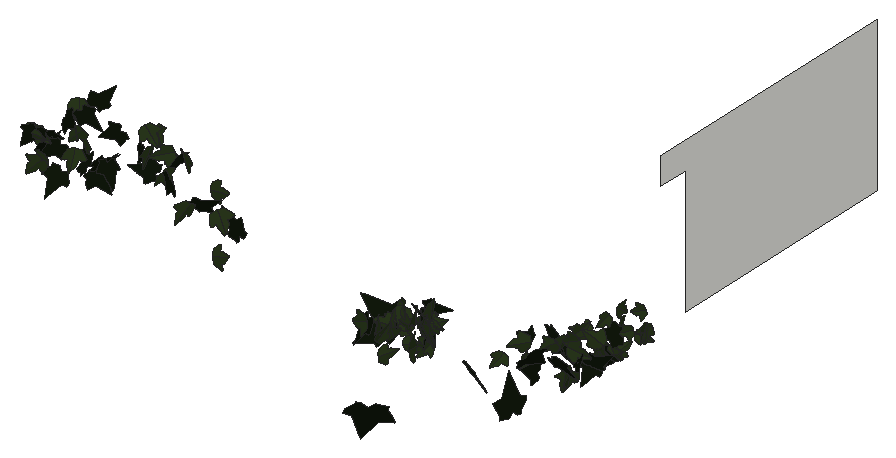
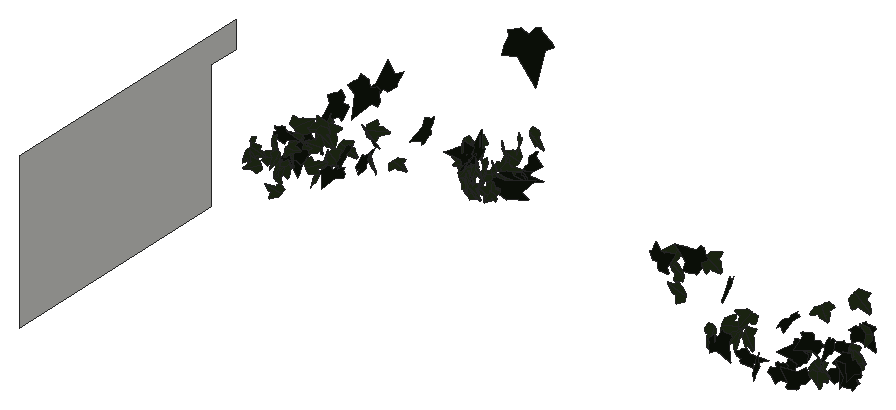
# SketchUp Ruby script. Lengths in inches.
U = 1.inch
M = Sketchup.active_model
def pt(a) = Geom::Point3d.new(a.map { |v| v * U })
def face(e, loops, mat)
  f = e.add_face(loops[0].map { |a| pt(a) })
  loops[1..].each { |l| e.add_face(l.map { |a| pt(a) }).erase! }
  f.material = f.back_material = mat if mat
  f
end
# faces: each face lists its corners as indices into pts; further lists are holes
def faces(e, pts, list, mat = nil) = list.each { |f| face(e, (f[0].is_a?(Array) ? f : [f]).map { |l| l.map { |i| pts[i] } }, mat) }
# xy, xz, yz: faces in a plane at the given z, y or x. An outline is a flat list of corners, or four numbers for a rectangle; further outlines are holes
def ring(l) = l.size == 4 ? [[l[0], l[1]], [l[2], l[1]], [l[2], l[3]], [l[0], l[3]]] : l.each_slice(2).to_a
def flat(e, list, mat, &to3) = list.each { |f| face(e, (f[0].is_a?(Array) ? f : [f]).map { |l| ring(l).map { |u, v| to3.(u, v) } }, mat) }
def xy(e, z, list, mat = nil) = flat(e, list, mat) { |x, y| [x, y, z] }
def xz(e, y, list, mat = nil) = flat(e, list, mat) { |x, z| [x, y, z] }
def yz(e, x, list, mat = nil) = flat(e, list, mat) { |y, z| [x, y, z] }
def lines(e, pts, list) = list.each { |a, b| e.add_line(pt(pts[a]), pt(pts[b])) }
# prism: a flat outline (further loops are holes) pulled along v
def prism(e, loops, v, mat = nil)
  f = face(e, loops, mat); d = Geom::Vector3d.new(v.map { |x| x * U })
  f.pushpull(f.normal.samedirection?(d) ? d.length : -d.length)
end
def box(e, o, s, mat = nil) = prism(e, [[o, [o[0] + s[0], o[1], o[2]], [o[0] + s[0], o[1] + s[1], o[2]], [o[0], o[1] + s[1], o[2]]]], [0, 0, s[2]], mat)
def at(x, y, z, deg = 0) = Geom::Transformation.translation(pt([x, y, z])) * Geom::Transformation.rotation(ORIGIN, Z_AXIS, deg.degrees)
def axes(o, x, y, z) = Geom::Transformation.new([*x, 0, *y, 0, *z, 0, *pt(o).to_a, 1])
def part(name) = M.definitions.add(name)
# library, detail: a bought-in or finely detailed component or shape, given as its bounding box
def library(name, o, s) = part(name).tap { |d| box(d.entities, o, s) }
def detail(e, o, s) = box(e.add_group.entities, o, s)
def put(e, d, t, mat = nil) = e.add_instance(d, t).tap { |i| i.material = mat if mat }
def group(e, t, mat = nil) = e.add_group.tap { |g| g.transformation = t; g.material = mat if mat }.entities
root = M.entities
M.materials.add("efeu1").color = [18, 25, 13]
M.materials.add("efeu2").color = [43, 57, 29]
c1 = part("ivyleaf_10")
p = [[0,0.5,-0.03],[-0.0625,2.02,-0.43],[-0.19,2.01,-0.46],[-0.54,1.05,-0.29],[-0.52,0.625,-0.18],[-0.83,0.76,-0.28],
  [-1.16,0.64,-0.33],[-1.15,0.33,-0.24],[-0.77,-0.39,0.02],[-0.3,-0.51,0.16],[0.04,-0.48,0.23],[-0.02,2.01,-0.4375],
  [-0.06,2.01,-0.43],[0.04,-0.49,0.23],[0.67,-0.49,0.14],[1.38,0.36,-0.2],[1.375,0.51,-0.24],[0.81,0.65,-0.19],
  [0.62,0.59,-0.15],[0.6,1.09,-0.28],[0.5,1.23,-0.31]]
faces(c1.entities,p,[[0,1,2,3,4,5,6,7,8,9,10],[11,12,0,13,14,15,16,17,18,19,20]],"efeu2")
c2 = part("ivyleaf_9")
p = [[1.54,2.16,1.25],[1.36,2.04,1.19],[-0.21,0.99,0.68],[-0.71,1.11,0.82],[-0.85,0.86,0.67],[-0.8,0.17,0.21],
  [-0.9,-0.01,0.1],[-0.67,-0.16,-0.02],[-0.08,-0.08,-0.05],[-0.03,-0.6,-0.4],[0.65,-0.88,-0.66],[0.83,-0.6,-0.49],
  [1.29,-0.42,-0.43],[1.8125,-0.07,-0.26],[1.21,0.44,0.15]]
faces(c2.entities,p,[[0,1,2,3,4,5,6,7,8,9,10,11,12,13,14]],"efeu1")
p = [[600,172.6875,154.12],[600,172.6875,171.1],[600.49,142.28,171.1],[600.49,142.28,168.16],[600.44,145.72,168.16],[600.44,145.72,154.12]]
faces(root,p,[[0,1,2,3,4,5]])
put(root,c1,axes([538.16,133.79,155.21],[0.18163,0.01122,0.75224],[0.73526,0.16121,-0.17993],[-0.1593,0.75687,0.02717]))
put(root,c2,axes([538.4,134.09,153.71],[0.30381,0.77459,-0.0565],[-0.01137,0.06509,0.83133],[0.77656,-0.30209,0.03427]))
put(root,c1,axes([538.64,138.9,156.16],[0.7212,0.27698,0.03221],[0.02999,0.01177,-0.77256],[-0.27723,0.72182,0.00023]))
put(root,c2,axes([538.86,134.06,155.24],[0.69763,0.51598,-0.17397],[-0.14038,-0.10277,-0.86772],[-0.52612,0.71162,0.00083]))
put(root,c2,axes([539.65,131.65,157.125],[0.19614,0.36038,-0.73019],[-0.34317,-0.64453,-0.41029],[-0.73844,0.39526,-0.00328]))
put(root,c2,axes([539.93,134.62,154.3],[0.02323,0.06156,-0.80436],[-0.30244,-0.74534,-0.06577],[-0.74788,0.30332,0.00162]))
put(root,c1,axes([539.03,131.61,156.8],[-0.18917,0.06706,-0.77238],[0.75356,-0.17103,-0.1994],[-0.18229,-0.7766,-0.02279]))
put(root,c2,axes([539.55,140.36,155.67],[-0.19047,-0.10209,0.79318],[0.77188,0.18982,0.20979],[-0.2092,0.79334,0.05188]))
put(root,c1,axes([540.03,136.89,154.5],[-0.51647,0.40191,0.41635],[0.33105,-0.25253,0.65441],[0.47464,0.61345,-0.00339]))
put(root,c1,axes([540.78,131.4,154.4375],[0.30694,-0.14086,-0.77767],[-0.71473,0.30658,-0.33763],[0.33731,0.77781,-0.00775]))
put(root,c2,axes([540.38,135.1,157],[0.17453,-0.20926,-0.75548],[-0.52984,0.53894,-0.27169],[0.57776,0.55746,-0.02094]))
put(root,c1,axes([540.8125,136.42,155.11],[-0.53976,-0.24221,0.56706],[-0.51907,-0.22834,-0.59161],[0.33286,-0.74884,-0.00302]))
put(root,c2,axes([541.37,136.16,157.42],[-0.0648,-0.13453,-0.80919],[0.55258,0.59275,-0.1428],[0.60625,-0.55465,0.04366]))
put(root,c2,axes([543.28,138.8,155.03],[-0.03916,0.10134,-0.79983],[-0.5954,-0.54355,-0.03972],[-0.54359,0.58805,0.10112]))
put(root,c2,axes([542.9,131,154.14],[-0.68653,-0.5213,-0.0395],[0.03659,0.01712,-0.86198],[0.52152,-0.68746,0.00848]))
put(root,c1,axes([543.51,127.41,157.07],[-0.55173,-0.34553,0.61966],[-0.503,-0.3631,-0.65033],[0.50036,-0.74602,0.02952]))
put(root,c1,axes([543.25,134.12,155.76],[-0.53137,0.47422,-0.42591],[0.30278,-0.30016,-0.71195],[-0.5609,-0.61128,0.01917]))
put(root,c2,axes([544.21,133.08,154.47],[-0.63931,0.2044,-0.45949],[-0.43596,0.14522,0.67118],[0.2507,0.7738,-0.00459]))
put(root,c2,axes([544.41,136.02,153.72],[-0.33925,0.575,-0.45103],[0.20796,-0.40075,-0.66731],[-0.70058,-0.3974,0.02033]))
put(root,c2,axes([544.52,133.79,154.14],[0.05579,0.62679,-0.58324],[-0.04631,0.58583,0.62515],[0.85492,-0.00917,0.07192]))
put(root,c1,axes([544.81,130.57,156.96],[0.56058,0.63253,-0.23032],[-0.15906,-0.16677,-0.84515],[-0.65409,0.58265,0.00813]))
put(root,c2,axes([545.01,133.38,153.82],[0.03779,-0.50189,-0.72315],[-0.05962,0.72069,-0.5033],[0.87823,0.07052,-0.00306]))
put(root,c2,axes([545.875,138.52,154.37],[-0.02382,0.00622,-0.82368],[0.71569,-0.40778,-0.02378],[-0.40777,-0.71606,0.00638]))
put(root,c2,axes([547.1,132.48,155.89],[0.04586,-0.77951,-0.22466],[-0.01365,0.22425,-0.78086],[0.81112,0.04784,-0.00044]))
put(root,c1,axes([547.72,138.49,156.72],[-0.15617,0.81876,0.06978],[-0.01288,0.06859,-0.83352],[-0.82162,-0.1567,-0.0002]))
put(root,c2,axes([548.48,137,153.48],[-0.38187,0.07115,0.73811],[-0.72908,0.11553,-0.38833],[-0.13536,-0.82298,0.0093]))
put(root,c1,axes([548.23,136.72,155.76],[0.12811,-0.82101,0.27076],[0.07379,-0.26233,-0.83037],[0.86135,0.14458,0.03086]))
put(root,c1,axes([548.08,136.63,157.75],[0.59729,0.41037,0.48709],[0.37733,0.30997,-0.72385],[-0.51311,0.70564,0.03469]))
put(root,c1,axes([550.34,136.91,156.13],[0.16305,0.08602,-0.82421],[-0.70824,-0.42167,-0.18411],[-0.43025,0.72671,-0.00927]))
put(root,c2,axes([550.38,138,155.27],[-0.07722,0.63035,-0.56912],[0.09084,-0.56206,-0.63485],[-0.84438,-0.11811,-0.01626]))
put(root,c1,axes([550.95,135.43,154.9],[-0.31424,-0.69836,-0.44569],[0.19447,0.40118,-0.76573],[0.80532,-0.36938,0.01099]))
put(root,c1,axes([551.18,137.97,155.75],[-0.7459,0.42304,-0.01831],[0.01592,-0.00904,-0.85751],[-0.42314,-0.74607,0.00001]))
put(root,c2,axes([553.61,132.75,156.47],[0.4271,-0.24571,-0.70668],[0.60894,-0.35862,0.49272],[-0.4347,-0.74378,-0.00412]))
put(root,c1,axes([557.17,134.7,155.82],[0.12973,-0.0419,-0.87246],[0.81019,-0.32381,0.13602],[-0.32638,-0.82046,-0.00913]))
put(root,c1,axes([558.06,129.68,156.66],[-0.22354,-0.67295,0.54403],[-0.10724,-0.53601,-0.70709],[0.85867,-0.24213,0.05332]))
put(root,c2,axes([558.53,130.5,156.67],[0.64407,0.48312,-0.40607],[0.32501,0.24344,0.80513],[0.54099,-0.72143,-0.00025]))
put(root,c1,axes([561.23,130.13,156.78],[0.52281,0.70498,0.2678],[0.16092,0.21407,-0.87768],[-0.73676,0.54701,-0.00166]))
put(root,c2,axes([562.92,130.68,155.23],[0.0634,-0.10933,0.99298],[-0.68294,0.72142,0.12303],[-0.72908,-0.68527,-0.0289]))
put(root,c1,axes([562.01,128.83,153.5],[0.28453,-0.18791,-0.84865],[0.74938,-0.39941,0.33969],[-0.4404,-0.80103,0.02971]))
put(root,c2,axes([582.43,127.95,154.38],[-1.0884,-0.64831,-0.54177],[-0.43949,-0.32015,1.26602],[-0.72158,1.17288,0.0461]))
put(root,c2,axes([581.74,125.07,155.83],[-0.02417,-0.01205,-0.91198],[0.56003,-0.72025,-0.00532],[-0.71987,-0.55993,0.02647]))
put(root,c2,axes([582.35,125.81,154.49],[-0.59916,-0.32383,0.4931],[-0.42255,-0.25486,-0.68081],[0.41165,-0.73293,0.01887]))
put(root,c2,axes([583.1,126.6,154.76],[-0.5473,0.0676,0.53336],[-0.53523,0.0033,-0.54963],[-0.05073,-0.7642,0.04481]))
put(root,c1,axes([582.99,126.52,155.14],[0.14239,0.17184,0.74485],[-0.56321,-0.4887,0.22041],[0.51685,-0.57987,0.03498]))
put(root,c1,axes([583.14,122.71,157.2],[0.32433,-0.22794,-0.81599],[-0.67575,0.45743,-0.39637],[0.51104,0.74952,-0.00626]))
put(root,c1,axes([582.91,128.51,155.63],[0.61668,0.31527,-0.16842],[-0.15247,-0.07174,-0.69258],[-0.32328,0.63523,0.00537]))
put(root,c1,axes([582.67,128.54,156.21],[0.39763,-0.1483,0.61159],[0.57181,-0.21699,-0.42437],[0.26281,0.69646,-0.00199]))
put(root,c1,axes([583.14,128.62,154.11],[0.63031,0.27778,0.07534],[-0.07011,-0.02772,0.6888],[0.27915,-0.63419,0.00289]))
put(root,c1,axes([584,127.84,154.95],[-0.07099,-0.01051,0.63782],[-0.63754,0.02298,-0.07058],[-0.02168,-0.64134,-0.01299]))
put(root,c1,axes([583.2,128.58,153.99],[0.54948,0.03532,0.39755],[0.39654,0.02841,-0.55061],[-0.04527,0.67762,0.00236]))
put(root,c1,axes([583.68,124.12,156.7],[-0.04347,0.20265,-0.74578],[0.20959,-0.71587,-0.20674],[-0.74386,-0.21355,-0.01467]))
put(root,c1,axes([583.86,124.21,155.14],[0.01918,-0.59675,0.48372],[-0.02502,0.48313,0.59701],[-0.76777,-0.03065,-0.00737]))
put(root,c1,axes([584.06,125.75,154.84],[-0.24294,-0.54044,-0.26284],[-0.10862,-0.23935,0.59253],[-0.59107,0.26611,-0.00086]))
put(root,c1,axes([583.93,125.62,156.16],[0.46115,-0.45321,-0.14519],[0.10334,-0.10198,0.64657],[-0.46454,-0.47258,-0.00029]))
put(root,c1,axes([584.01,124.29,153.46],[0.04693,0.03629,-0.77118],[0.48642,0.59857,0.05777],[0.59952,-0.4885,0.01349]))
put(root,c1,axes([583.98,127.6875,153.0625],[0.18511,-0.01668,-0.62513],[0.62378,-0.04121,0.18581],[-0.04425,-0.65065,0.00425]))
put(root,c1,axes([585.65,128.02,155.49],[-0.15905,0.07464,0.7275],[-0.72612,0.07245,-0.16619],[-0.087,-0.74115,0.05702]))
put(root,c1,axes([585.32,128.61,155.57],[0.08297,0.81543,0.03993],[0.00051,0.04008,-0.81964],[-0.81641,0.08289,0.00354]))
put(root,c1,axes([585.74,128.16,152.92],[-0.2941,-0.21841,-0.59072],[-0.43307,-0.40324,0.3647],[-0.45728,0.52235,0.03453]))
put(root,c1,axes([585.67,128.5,155.34],[-0.13623,-0.6718,0.17915],[-0.03624,-0.17545,-0.68547],[0.69433,-0.14096,-0.00063]))
put(root,c1,axes([585.78,128.86,154.98],[0.32065,-0.5272,-0.54501],[-0.24253,0.48934,-0.61604],[0.71844,0.40049,0.03529]))
put(root,c1,axes([586,128.2,153.57],[0.57919,-0.07349,-0.5641],[-0.56073,0.06187,-0.58379],[0.09584,0.80612,-0.00662]))
put(root,c2,axes([585.51,127.77,156.46],[0.68865,-0.41895,0.0137],[-0.00933,0.01102,0.80606],[-0.41907,-0.68869,0.00457]))
put(root,c1,axes([585.79,128.8,154.26],[0.21944,-0.40296,0.44391],[-0.20222,0.39527,0.45877],[-0.5644,-0.29829,0.00823]))
put(root,c1,axes([586.14,125.67,154.15],[-0.16725,0.25846,0.9999],[-0.62411,0.78175,-0.30647],[-0.82285,-0.64547,0.02921]))
put(root,c2,axes([585.71,128.46,155.34],[-0.45159,0.13948,-0.60683],[0.5863,-0.15716,-0.47243],[-0.20965,-0.73992,-0.01405]))
put(root,c1,axes([585.99,126.3,157.33],[0.20387,-0.72268,-0.40395],[-0.07905,0.39712,-0.75036],[0.82413,0.21686,0.02796]))
put(root,c1,axes([585.5625,128.41,155.63],[0.55354,-0.34275,-0.36001],[0.30334,-0.19393,0.65105],[-0.39378,-0.6312,-0.00454]))
put(root,c2,axes([585.64,128.72,156.2],[0.22363,-0.78028,-0.04672],[-0.01099,0.04545,-0.8117],[0.7816,0.22389,0.00196]))
put(root,c1,axes([585.97,128.05,156.18],[-0.01333,-0.58735,-0.37432],[-0.01395,-0.37408,0.58748],[-0.69635,0.01874,-0.0046]))
put(root,c1,axes([586.2,128.48,155.34],[0.4409,-0.62792,-0.1945],[-0.09041,0.17405,-0.76684],[0.65111,0.44937,0.02523]))
put(root,c2,axes([585.62,128.45,157],[0.28689,0.25864,-0.69154],[0.39539,0.57274,0.37824],[0.62353,-0.48218,0.07834]))
put(root,c1,axes([585.94,128.37,154.8],[0.55403,-0.0658,0.45345],[0.45422,-0.01476,-0.55711],[0.06029,0.71579,0.0302]))
put(root,c1,axes([586.25,128.45,155.5],[-0.05708,-0.74506,0.32088],[0.24987,-0.32218,-0.70363],[0.77178,0.04921,0.25154]))
put(root,c1,axes([586.17,127.41,155.51],[-0.77043,0.3036,-0.33668],[0.31545,-0.11779,-0.82807],[-0.3256,-0.83249,-0.00562]))
put(root,c1,axes([585.91,128.08,156.05],[-0.41829,-0.05001,-0.71688],[0.71582,0.04413,-0.42075],[0.06335,-0.82881,0.02085]))
put(root,c1,axes([586.41,127.98,157.6],[0.11015,-0.83784,-0.05423],[0.14336,0.07266,-0.8314],[0.82726,0.09897,0.1513]))
put(root,c1,axes([585.88,128.15,156.04],[-0.25597,0.07274,-0.78004],[0.74751,-0.22292,-0.26609],[-0.23447,-0.79012,0.00326]))
put(root,c1,axes([586.17,127.53,155.69],[-0.58845,0.42957,-0.50643],[0.41564,-0.28949,-0.72851],[-0.51793,-0.72038,-0.00923]))
put(root,c1,axes([586.42,128.07,155.86],[0.24097,-0.00754,-0.7329],[0.73156,0.04976,0.24002],[0.04492,-0.76989,0.02269]))
put(root,c1,axes([592.85,129.7,154.09],[0.41934,0.29402,-0.45726],[-0.37046,-0.26808,-0.51212],[-0.39786,0.55951,-0.00509]))
put(root,c2,axes([593.68,110.21,157.6875],[0.6731,1.01451,-0.90267],[-0.52693,-0.73341,-1.21719],[-1.25155,0.85439,0.027]))
put(root,c2,axes([593.01,124.9,155.22],[0.78297,-0.52366,0.08494],[0.07891,-0.03478,-0.94183],[0.5246,0.7868,0.0149]))
put(root,c1,axes([594.56,130.59,153.34],[0.66799,-0.44559,-0.00085],[0.00659,0.00835,0.8029],[-0.44554,-0.66793,0.0106]))
put(root,c2,axes([595.47,130.17,156.13],[-0.30986,0.44803,0.63832],[-0.40859,0.49178,-0.54351],[-0.66426,-0.51149,0.03656]))
put(root,c1,axes([595.49,129.76,156.38],[-0.09704,-0.06481,0.81421],[-0.43252,-0.69146,-0.10659],[0.69287,-0.44072,0.0475]))
put(root,c2,axes([595.16,133.71,155.76],[0.59007,-0.6358,0.02525],[0.02337,-0.01276,-0.86738],[0.63587,0.59047,0.00845]))
put(root,c2,axes([595.83,130.83,153.02],[-0.107,-0.05321,0.83212],[-0.37444,-0.74653,-0.09589],[0.74502,-0.38285,0.07132]))
put(root,c1,axes([596.57,132.18,155.49],[-0.36148,-0.24223,0.61925],[-0.50422,-0.35964,-0.43502],[0.43349,-0.62032,0.0104]))
put(root,c2,axes([595.84,134.64,154.48],[-0.14012,-0.56673,-0.59091],[0.14984,0.57163,-0.58376],[0.80492,-0.20507,0.00581]))
put(root,c1,axes([596.59,133.84,155.28],[-0.09509,-0.58735,0.38305],[-0.05692,-0.37882,-0.59499],[0.69891,-0.11077,0.00366]))
put(root,c1,axes([597.02,136.31,155.07],[0.15515,0.21267,0.71147],[-0.41438,-0.57834,0.26324],[0.6162,-0.44247,-0.00211]))
put(root,c1,axes([597.36,133.95,154.12],[-0.42331,0.60693,0.02947],[0.0098,-0.02909,0.73991],[0.60756,0.42333,0.00859]))
put(root,c1,axes([597.45,135.27,152.99],[-0.20029,0.62397,0.045],[0.00865,-0.04448,0.65531],[0.62553,0.2004,0.00535]))
put(root,c1,axes([597.62,134.4,156.07],[-0.09216,-0.40307,0.54853],[0.11465,0.53643,0.41345],[-0.67097,0.14702,-0.00469]))
put(root,c1,axes([598.73,132.69,156.15],[0.31836,-0.07905,-0.86369],[-0.78248,0.37064,-0.32235],[0.37407,0.84258,0.06076]))
put(root,c1,axes([598.66,137.05,156.72],[0.176,0.29213,-0.54169],[-0.28469,-0.46085,-0.34103],[-0.54563,0.33469,0.00321]))
put(root,c1,axes([598.61,138.9,156.76],[-0.00365,0.3676,0.57838],[-0.19795,0.55317,-0.35283],[-0.6561,-0.16894,0.10323]))
put(root,c2,axes([598.8,125.87,157.67],[0.46039,0.96467,0.33598],[0.11899,0.31537,-1.06856],[-1.01455,0.47474,0.02714]))
put(root,c1,axes([598.79,136.49,155.23],[0.05785,-0.07394,0.6497],[0.56506,-0.32258,-0.08702],[0.32906,0.56692,0.03522]))
put(root,c1,axes([598.87,138.37,152.89],[0.34082,0.20985,-0.55696],[0.48556,0.27314,0.40004],[0.3442,-0.59309,-0.01284]))
put(root,c2,axes([599.25,132.03,154.24],[-0.12092,0.37533,0.76142],[0.23364,-0.72469,0.39433],[0.81612,0.26308,-0.00008]))
put(root,c1,axes([599.18,131.59,156.12],[0.19228,0.07049,0.84959],[0.74407,0.41121,-0.20252],[-0.41609,0.76791,0.03045]))
put(root,c1,axes([600.22,136.9,153.54],[-0.41408,0.3247,-0.50915],[-0.42609,0.28038,0.52533],[0.42793,0.59337,0.03039]))
put(root,c1,axes([599.87,135.96,153.99],[-0.08974,-0.24113,-0.73636],[0.23716,0.69716,-0.25719],[0.73765,-0.25347,-0.0069]))
put(root,c1,axes([600.45,137.9375,155.66],[0.1757,0.08984,-0.6067],[-0.56838,-0.21326,-0.19619],[-0.23043,0.59454,0.02131]))
put(root,c1,axes([600.33,129.88,154.75],[-0.48408,-0.72056,0.30516],[-0.15204,-0.26539,-0.86782],[0.7676,-0.50698,0.02056]))
put(root,c2,axes([599.8,134.11,154.9],[0.03655,0.07425,-0.7763],[0.14635,0.7627,0.07984],[0.76599,-0.14926,0.02179]))
put(root,c1,axes([600.62,133.43,156.58],[0.42321,0.31993,0.69004],[-0.55902,-0.40463,0.53045],[0.51576,-0.70109,0.00874]))
put(root,c1,axes([600.64,139.49,157.07],[0.26276,-0.07589,-0.57907],[-0.56642,0.12164,-0.27295],[0.14233,0.62416,-0.01722]))
put(root,c1,axes([600.1875,137.41,156.9375],[0.291,-0.51907,0.28916],[0.14392,-0.25081,-0.59507],[0.57648,0.32464,0.00259]))
put(root,c1,axes([600.25,133.53,154.16],[-0.66859,-0.38271,0.12977],[0.12044,0.05075,0.77022],[-0.38575,0.67917,0.01557]))
put(root,c1,axes([600.4,134.78,155.29],[0.18212,0.50974,-0.49504],[-0.20666,-0.45095,-0.54037],[-0.67985,0.27364,0.03165]))
put(root,c2,axes([600.54,133.85,154.34],[0.14671,0.71595,-0.25118],[-0.06054,-0.24397,-0.73076],[-0.75632,0.15841,0.00977]))
put(root,c2,axes([600.43,132.99,154.52],[-0.35798,-0.69155,0.18575],[-0.08783,-0.1637,-0.7787],[0.71065,-0.36858,-0.00267]))
put(root,c1,axes([600.52,133.33,155.27],[-0.00228,0.33527,0.71812],[-0.22748,0.68763,-0.32175],[-0.75918,-0.20705,0.09425]))
put(root,c2,axes([599.97,128.22,156.78],[0.96204,0.02659,0.05862],[0.05863,0.0003,-0.9624],[-0.02656,0.96382,-0.00132]))
put(root,c2,axes([600.68,121.39,155.17],[-0.52006,-0.81045,0.65983],[0.5208,0.43799,0.94846],[-0.90607,0.71694,0.16645]))
put(root,c2,axes([601.24,135.4,156.71],[-0.24385,-0.21141,-0.71782],[-0.57855,-0.42556,0.32187],[-0.4746,0.6274,-0.02356]))
put(root,c1,axes([600.3,129.73,154.85],[0.02424,-0.06206,0.92116],[0.55328,-0.73671,-0.06419],[0.73911,0.55352,0.01784]))
put(root,c2,axes([600.46,132.73,154.5625],[0.07067,-0.09791,0.79975],[0.80415,0.0587,-0.06388],[-0.05031,0.80072,0.10247]))
put(root,c1,axes([600.85,138.76,154.99],[0.15509,0.12201,0.62426],[0.48856,0.3886,-0.19733],[-0.40731,0.51258,0.00101]))
put(root,c1,axes([601.65,138.74,155.71],[-0.40366,-0.50379,0.07924],[0.03438,-0.12771,-0.63682],[0.50882,-0.39104,0.10589]))
put(root,c1,axes([601.71,138.7,156.05],[-0.20686,-0.62156,0.06595],[0.07571,-0.09387,-0.64725],[0.62045,-0.19578,0.10097]))
put(root,c1,axes([601.95,138.15,156.5],[0.29926,-0.54013,0.29558],[0.17311,-0.24158,-0.61672],[0.59089,0.34433,0.03097]))
